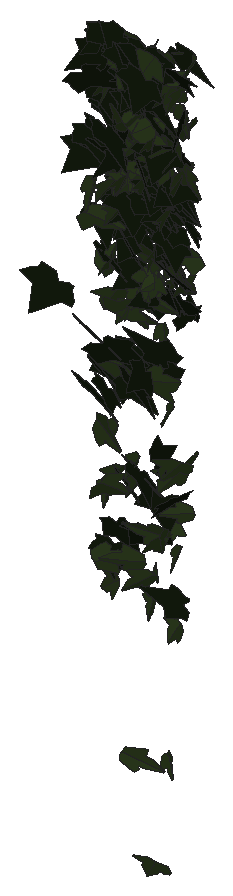
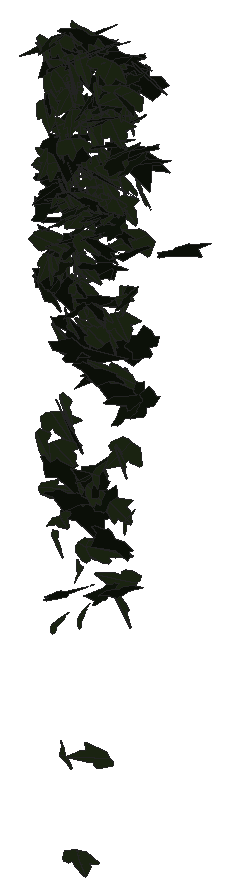
# SketchUp Ruby script. Lengths in millimetres.
U = 1.mm
M = Sketchup.active_model
def pt(a) = Geom::Point3d.new(a.map { |v| v * U })
def face(e, loops, mat)
  f = e.add_face(loops[0].map { |a| pt(a) })
  loops[1..].each { |l| e.add_face(l.map { |a| pt(a) }).erase! }
  f.material = f.back_material = mat if mat
  f
end
# faces: each face lists its corners as indices into pts; further lists are holes
def faces(e, pts, list, mat = nil) = list.each { |f| face(e, (f[0].is_a?(Array) ? f : [f]).map { |l| l.map { |i| pts[i] } }, mat) }
# xy, xz, yz: faces in a plane at the given z, y or x. An outline is a flat list of corners, or four numbers for a rectangle; further outlines are holes
def ring(l) = l.size == 4 ? [[l[0], l[1]], [l[2], l[1]], [l[2], l[3]], [l[0], l[3]]] : l.each_slice(2).to_a
def flat(e, list, mat, &to3) = list.each { |f| face(e, (f[0].is_a?(Array) ? f : [f]).map { |l| ring(l).map { |u, v| to3.(u, v) } }, mat) }
def xy(e, z, list, mat = nil) = flat(e, list, mat) { |x, y| [x, y, z] }
def xz(e, y, list, mat = nil) = flat(e, list, mat) { |x, z| [x, y, z] }
def yz(e, x, list, mat = nil) = flat(e, list, mat) { |y, z| [x, y, z] }
def lines(e, pts, list) = list.each { |a, b| e.add_line(pt(pts[a]), pt(pts[b])) }
# prism: a flat outline (further loops are holes) pulled along v
def prism(e, loops, v, mat = nil)
  f = face(e, loops, mat); d = Geom::Vector3d.new(v.map { |x| x * U })
  f.pushpull(f.normal.samedirection?(d) ? d.length : -d.length)
end
def box(e, o, s, mat = nil) = prism(e, [[o, [o[0] + s[0], o[1], o[2]], [o[0] + s[0], o[1] + s[1], o[2]], [o[0], o[1] + s[1], o[2]]]], [0, 0, s[2]], mat)
def at(x, y, z, deg = 0) = Geom::Transformation.translation(pt([x, y, z])) * Geom::Transformation.rotation(ORIGIN, Z_AXIS, deg.degrees)
def axes(o, x, y, z) = Geom::Transformation.new([*x, 0, *y, 0, *z, 0, *pt(o).to_a, 1])
def part(name) = M.definitions.add(name)
# library, detail: a bought-in or finely detailed component or shape, given as its bounding box
def library(name, o, s) = part(name).tap { |d| box(d.entities, o, s) }
def detail(e, o, s) = box(e.add_group.entities, o, s)
def put(e, d, t, mat = nil) = e.add_instance(d, t).tap { |i| i.material = mat if mat }
def group(e, t, mat = nil) = e.add_group.tap { |g| g.transformation = t; g.material = mat if mat }.entities
root = M.entities
M.materials.add("efeu1").color = [18, 25, 13]
M.materials.add("efeu2").color = [43, 57, 29]
c1 = part("ivyleaf_9")
p = [[39.1,54.8,31.7],[34.5,51.8,30.2],[-5.3,25.2,17.3],[-17.9,28.3,20.9],[-21.6,21.7,17],[-20.2,4.3,5.3],
  [-22.9,-0.3,2.5],[-17.1,-4,-0.6],[-2,-2.1,-1.2],[-0.7,-15.4,-10.1],[16.6,-22.3,-16.7],[21.1,-15.1,-12.5],
  [32.7,-10.7,-11],[46.1,-1.8,-6.6],[30.8,11.2,3.8]]
faces(c1.entities,p,[[0,1,2,3,4,5,6,7,8,9,10,11,12,13,14]],"efeu1")
c2 = part("ivyleaf_10")
p = [[0,12.8,-0.8],[-1.5,51.3,-10.9],[-4.9,51,-11.6],[-13.6,26.5,-7.3],[-13.2,15.9,-4.6],[-21.1,19.3,-7.2],
  [-29.5,16.3,-8.3],[-29.2,8.3,-6.2],[-19.7,-9.8,0.5],[-7.6,-13,4],[1,-12.2,5.8],[-0.4,51.1,-11.1],
  [-1.5,51.1,-10.9],[1,-12.4,5.9],[16.9,-12.4,3.5],[35.1,9.1,-5.1],[35,12.9,-6.1],[20.5,16.4,-4.9],
  [15.8,15,-3.8],[15.3,27.6,-7.1],[12.8,31.3,-7.8]]
faces(c2.entities,p,[[0,1,2,3,4,5,6,7,8,9,10],[11,12,0,13,14,15,16,17,18,19,20]],"efeu2")
put(root,c1,axes([1383.5,966.4,1257.2],[-0.18565,-0.81237,-0.03715],[-0.00199,0.03754,-0.81819],[1.54772,-0.09739,-0.00551]))
put(root,c1,axes([1375.5,982.3,1174.7],[0.78322,-0.66558,-0.0595],[-0.06187,0.04986,-0.78253],[1.27028,0.41281,-0.00143]))
put(root,c2,axes([1392.2,961.8,1154.5],[0.19233,0.43423,-0.7713],[0.2857,0.75665,0.44565],[1.66017,-0.18052,0.01266]))
put(root,c1,axes([1404.6,919.2,1408.9],[-1.08984,-0.55615,0.3063],[-0.4056,-0.22018,-0.79821],[1.13828,-0.61094,0.00884]))
put(root,c1,axes([1401.9,817.4,1189],[-0.98408,-0.7657,0.35319],[-0.37558,-0.29292,-0.92393],[1.56027,-0.55344,0.00036]))
put(root,c1,axes([1390.4,991.5,581.7],[-0.42642,-0.73146,-0.03867],[0.02209,0.03689,-0.76501],[1.39389,-0.22435,0.00029]))
put(root,c1,axes([1381.2,961.4,1429.5],[0.25074,-0.76568,0.26519],[0.03916,-0.26543,-0.77658],[1.54168,0.13127,-0.0234]))
put(root,c1,axes([1413.5,922.4,1607.9],[-1.48911,0.25969,-0.15704],[0.25456,-0.09474,-0.82306],[-0.51847,-0.79239,0.04694]))
put(root,c1,axes([1388.4,976.2,1599.5],[-0.33598,-0.66441,0.46982],[0.06722,-0.48655,-0.6748],[1.54725,-0.12314,0.13134]))
put(root,c2,axes([1403.1,984.2,740.7],[-0.16619,-0.65374,0.43706],[-0.0428,-0.43749,-0.65888],[1.49603,-0.08514,0.0297]))
put(root,c2,axes([1404.7,989.4,1515.6],[-0.62529,-0.70465,0.21746],[-0.00263,-0.23747,-0.7716],[1.40349,-0.31439,0.09544]))
put(root,c2,axes([1403,962.3,1167.3],[0.01424,-0.65222,-0.3851],[0.01668,0.38517,-0.65217],[1.44144,0.00199,0.01135]))
put(root,c1,axes([1386.3,983.2,1464.5],[0.0237,-0.7808,0.15686],[0.08453,-0.15596,-0.77982],[1.51335,0.02094,0.0411]))
put(root,c2,axes([1390.4,970.3,707.1],[-0.11612,-0.33846,0.66501],[0.68804,-0.5971,-0.27073],[1.24234,0.29906,0.21209]))
put(root,c2,axes([1384.8,976.6,1581.2],[-1.09415,-0.2681,-0.53427],[1.02316,0.09222,-0.62475],[0.49743,-0.77939,0.10986]))
put(root,c2,axes([1401.6,954,1527.8],[-0.08183,-0.71014,-0.39764],[0.15773,0.3923,-0.70957],[1.54094,-0.07787,0.05151]))
put(root,c1,axes([1380.6,952.1,962.6],[1.11983,-0.58371,-0.01156],[-0.00828,0.01203,-0.82879],[1.11111,0.58838,0.00548]))
put(root,c1,axes([1421.5,957.3,1591.2],[0.00068,0.82514,0.02135],[-0.27759,0.02107,-0.81216],[-1.54622,-0.00342,0.14581]))
put(root,c2,axes([1414.1,964,1109.5],[-0.74767,-0.6209,0.19031],[-0.12579,-0.18304,-0.73362],[1.22955,-0.39629,0.04067]))
put(root,c2,axes([1388.3,932.7,1268.5],[-0.64985,-0.38676,-0.75955],[1.19277,0.44065,-0.50611],[1.09947,-0.70664,0.10012]))
put(root,c1,axes([1393.6,955.9,1511.8],[0.11622,-0.80177,-0.0838],[0.00596,0.08428,-0.80404],[1.53423,0.06041,0.00947]))
put(root,c1,axes([1380.9,929.1,927.7],[0.64459,-0.71847,0.40917],[0.42658,-0.34582,-0.79277],[1.51466,0.40315,0.04914]))
put(root,c1,axes([1379.7,923.7,1046.8],[0.85251,-0.55382,0.40403],[0.50513,-0.3049,-0.71218],[1.20296,0.52051,0.01272]))
put(root,c2,axes([1417.7,958.3,535.8],[0.71217,-0.58447,-0.45342],[-0.46518,0.3819,-0.694],[1.32877,0.44695,0.00006]))
put(root,c2,axes([1415.4,936.8,1528.4],[0.4615,-0.75581,-0.43029],[-0.22724,0.41354,-0.79368],[1.63957,0.27006,0.01111]))
put(root,c1,axes([1396.2,923.4,1440.7],[-0.05111,-0.77697,-0.22063],[0.04125,0.21998,-0.77732],[1.53665,-0.03175,0.01353]))
put(root,c2,axes([1413.2,962.8,836.9],[0.64822,-0.68731,-0.16805],[-0.09975,0.16149,-0.7667],[1.34293,0.34376,0.02417]))
put(root,c2,axes([1417,947.9,1333.2],[-0.13818,-0.73083,0.2927],[-0.08852,-0.28945,-0.73424],[1.4957,-0.08465,-0.01641]))
put(root,c1,axes([1423.3,914.8,1423],[0.81967,0.40867,-0.6231],[-0.81874,-0.45128,-0.59332],[-1.15799,0.60834,-0.02156]))
put(root,c1,axes([1400.2,960.7,912.8],[-0.01098,-0.62962,0.49023],[0.04838,-0.49014,-0.6292],[1.51791,0.01107,0.0236]))
put(root,c1,axes([1396.8,947.3,1583.9],[1.35766,-0.37155,-0.18742],[-0.17997,0.21749,-0.79108],[0.77128,0.70477,0.14532]))
put(root,c2,axes([1408.9,906.3,1349.8],[0.93175,-0.67898,0.4519],[0.50507,-0.36577,-0.83707],[1.46781,0.55687,0.00117]))
put(root,c1,axes([1397.3,984.5,1311.6],[0.96314,-0.58909,0.01522],[0.01538,-0.01313,-0.77661],[1.12143,0.50612,-0.00243]))
put(root,c1,axes([1406.8,952.5,1495],[-0.02656,-0.78957,0.17307],[-0.0277,-0.17282,-0.78961],[1.53813,-0.01675,-0.01123]))
put(root,c1,axes([1403.9,893.3,1573.3],[-0.03519,0.04954,-0.95837],[0.02758,0.95845,0.04927],[1.8262,-0.01352,-0.01921]))
put(root,c2,axes([1409.1,959.3,1397.8],[1.272,-0.50532,0.29755],[0.42359,-0.19882,-0.83757],[1.03257,0.70406,-0.02296]))
put(root,c1,axes([1437.9,951.7,1630.9],[-1.3885,-0.32156,0.24439],[-0.38375,-0.14723,-0.79565],[0.66604,-0.75519,0.05105]))
put(root,c2,axes([1399.4,949.9,576.1],[0.36962,0.17082,-0.85137],[1.22534,0.55707,0.25864],[1.10893,-0.67248,-0.00201]))
put(root,c1,axes([1407.8,950.8,1634.3],[-0.11101,-0.80044,-0.22127],[0.15875,0.21505,-0.79991],[1.57254,-0.07821,0.06513]))
put(root,c1,axes([1408.7,986.8,1406.1],[0.17531,-0.7858,-0.05674],[-0.00104,0.05706,-0.79115],[1.49942,0.09192,0.00608]))
put(root,c1,axes([1423.3,985,1469.4],[-0.76393,-0.64655,0.26374],[-0.14638,-0.26143,-0.75792],[1.32087,-0.4029,0.06854]))
put(root,c1,axes([1399,976.2,1438.8],[0.97484,-0.5797,0.21818],[0.25307,-0.1736,-0.77343],[1.15136,0.52898,-0.01472]))
put(root,c2,axes([1426.2,976.8,1623],[-1.51465,0.22786,-0.01391],[0.02986,0.00429,-0.82777],[-0.43343,-0.79595,-0.00844]))
put(root,c1,axes([1438.2,967.5,1294.5],[-1.54182,-0.05819,-0.14847],[0.28153,0.01297,-0.8122],[0.11339,-0.82351,-0.0023]))
put(root,c2,axes([1429.2,973.1,1080.6],[0.80247,-0.61306,-0.02625],[-0.01374,0.02689,-0.74401],[1.16777,0.4216,0.00928]))
put(root,c2,axes([1419.7,961.6,1407.7],[-0.37305,-0.80945,0.23875],[0.26558,0.21065,0.82873],[-1.58405,0.22594,0.08272]))
put(root,c2,axes([1437.3,969.2,1342],[-1.42296,0.22882,0.1356],[-0.23313,0.06288,-0.78153],[-0.44933,-0.75726,-0.02392]))
put(root,c2,axes([1439.3,948,1295.3],[-0.19729,-0.72072,0.30819],[-0.11005,-0.30299,-0.72802],[1.48776,-0.11798,-0.01298]))
put(root,c1,axes([1433.8,989.2,1518.9],[-0.77503,-0.65943,0.22641],[0.00689,-0.2642,-0.76297],[1.32692,-0.38379,0.1362]))
put(root,c1,axes([1424,979.1,1323.1],[-0.0649,-0.74925,-0.27158],[0.08543,0.26959,-0.74939],[1.51434,-0.04732,0.03064]))
put(root,c1,axes([1418.5,989.2,563.4],[0.61508,-0.69175,0.08443],[0.071,-0.07576,-0.76352],[1.32441,0.32532,0.00172]))
put(root,c1,axes([1442.1,989.7,1219.9],[-1.05635,-0.5197,-0.00477],[0.00635,0.00341,-0.76037],[0.98912,-0.55505,-0.00021]))
put(root,c1,axes([1431.3,958.3,968.4],[-1.04311,-0.38741,-0.45292],[0.77676,0.20444,-0.66876],[0.82662,-0.68098,0.05689]))
put(root,c2,axes([1436.5,967.7,1339.1],[1.1202,0.51681,-0.1362],[-0.18835,-0.0937,-0.78326],[-0.99959,0.59683,-0.00504]))
put(root,c1,axes([1469.6,981.4,1398.5],[-1.24986,0.35112,0.29934],[-0.64225,-0.0104,-0.72813],[-0.59887,-0.72165,0.15615]))
put(root,c2,axes([1450.7,971.8,1419],[-0.7007,-0.65439,0.27216],[-0.12306,-0.2744,-0.74724],[1.34323,-0.3665,0.07352]))
put(root,c1,axes([1429.8,971.7,1535.8],[-0.15257,-0.68111,0.44747],[0.2011,-0.45453,-0.67292],[1.53793,-0.00814,0.13238]))
put(root,c2,axes([1429.8,965.9,1075.1],[-1.17467,-0.4492,0.47082],[0.71501,0.28387,0.76333],[-1.01122,0.72252,-0.00719]))
put(root,c1,axes([1455,994.9,1149.8],[-1.07161,-0.4476,0.28525],[-0.38444,-0.20385,-0.7186],[0.93414,-0.59737,0.03149]))
put(root,c2,axes([1413.7,946.1,980.2],[0.10679,-0.03226,-0.86542],[1.58354,-0.23853,0.06284],[-0.45716,-0.83379,0.01551]))
put(root,c1,axes([1429.3,955.5,654.2],[-0.54245,-0.09388,-0.70569],[1.26493,0.23729,-0.30001],[0.4855,-0.72314,-0.00683]))
put(root,c1,axes([1430.4,973.5,733.9],[0.16223,-0.47252,0.60804],[0.28269,-0.59018,-0.47946],[1.43805,0.16932,0.02566]))
put(root,c1,axes([1464.3,991.5,1263.4],[-1.54721,-0.15313,-0.03686],[0.07134,0.00013,-0.82722],[0.29115,-0.81379,0.0068]))
put(root,c2,axes([1454.9,938.8,1361.2],[-0.04586,-0.79406,-0.01036],[0.00007,0.01036,-0.79442],[1.51138,-0.0241,-0.00028]))
put(root,c1,axes([1425.6,971.8,1222.1],[0.45769,-0.05898,-0.8232],[1.46631,-0.29137,0.24595],[-0.56316,-0.8066,-0.02865]))
put(root,c2,axes([1451.6,970.2,1345.4],[0.2024,-0.70765,0.32439],[0.21977,-0.30944,-0.71289],[1.46517,0.14417,0.06212]))
put(root,c2,axes([1462.4,953.6,1356.1],[-0.65566,-0.57467,0.50948],[-0.17857,-0.52271,-0.65304],[1.45069,-0.32407,0.14988]))
put(root,c1,axes([1456.5,970.9,1492.5],[-0.6835,-0.55118,0.48288],[-0.34395,-0.45452,-0.65322],[1.35155,-0.39441,0.07796]))
put(root,c1,axes([1449.4,980.5,1002.3],[-1.06445,-0.37036,-0.39864],[0.67013,0.18952,-0.67007],[0.78955,-0.66016,0.03128]))
put(root,c1,axes([1434.9,913.1,1031.9],[-0.06917,-0.04612,-0.91215],[0.5345,0.86808,-0.05508],[1.65401,-0.28245,-0.02034]))
put(root,c1,axes([1449.7,984.5,1274.2],[-0.33101,-0.77302,0.05514],[-0.00945,-0.0554,-0.79231],[1.47493,-0.17384,0.0073]))
put(root,c2,axes([1460.8,962.7,1558],[0.21322,-0.81799,-0.13795],[0.03213,0.14143,-0.82487],[1.57846,0.10762,0.03542]))
put(root,c2,axes([1453.6,972.3,781.9],[0.0192,-0.38628,0.67921],[0.42179,-0.64996,-0.37293],[1.42603,0.19744,0.10116]))
put(root,c2,axes([1477.3,906.4,1493.8],[-0.98023,0.32118,0.63002],[-1.00665,0.34237,-0.60694],[-0.89334,-0.73823,-0.00738]))
put(root,c1,axes([1437.2,984.1,1320.6],[0.28187,-0.75304,0.17605],[0.42696,-0.12971,-0.74354],[1.40854,0.19001,0.19015]))
put(root,c2,axes([1461.8,976.2,750.6],[-0.00776,-0.68886,0.41079],[0.03039,-0.41078,-0.68869],[1.52615,0.00468,0.0158]))
put(root,c2,axes([1454.7,975.6,1126],[1.32488,-0.36812,0.07239],[0.1193,-0.03632,-0.78747],[0.70399,0.69894,-0.00279]))
put(root,c1,axes([1436.2,939.2,1543],[0.76918,0.73771,-0.2474],[0.23254,0.21515,0.84115],[1.46248,-0.4222,-0.00363]))
put(root,c2,axes([1468.4,992.8,1267.4],[-0.46568,-0.60599,0.41848],[-0.13139,-0.42016,-0.64878],[1.39543,-0.24179,0.07857]))
put(root,c2,axes([1482.8,937.3,607.9],[-0.08652,-0.04195,0.78348],[-0.90717,-0.6219,-0.06095],[1.18611,-0.4787,0.01053]))
put(root,c2,axes([1483.1,988,1339.9],[-1.00138,-0.09019,0.55147],[-0.75997,-0.46919,-0.45772],[0.74397,-0.60069,0.27472]))
put(root,c2,axes([1440.6,983.9,1068.2],[-0.61494,-0.11608,0.7013],[1.33211,-0.18639,0.29163],[0.2361,0.74932,0.18118]))
put(root,c2,axes([1467.2,966.2,1469.8],[0.2262,-0.79103,0.21126],[0.10431,-0.20531,-0.79958],[1.55476,0.12886,0.02291]))
put(root,c1,axes([1453.9,930.4,1447.5],[0.06453,0.2424,0.91267],[-0.11875,-0.91069,0.24419],[1.79329,-0.06903,-0.01667]))
put(root,c2,axes([1466.4,963.3,1374.5],[0.74133,0.64995,-0.26409],[-0.28313,-0.21867,-0.7576],[-1.30483,0.41671,0.01435]))
put(root,c1,axes([1479.4,895.2,1436.2],[-1.25679,0.45424,-0.35024],[0.56807,-0.18394,-0.80134],[-0.9322,-0.7245,-0.01614]))
put(root,c1,axes([1456.2,981.6,1511.3],[0.31894,-0.77335,-0.15333],[-0.06192,0.14984,-0.7913],[1.49922,0.17071,-0.00006]))
put(root,c2,axes([1491.9,972.8,1199.9],[0.48907,-0.07163,-0.74482],[-1.01523,0.53472,-0.23547],[0.99865,0.57867,0.12538]))
put(root,c1,axes([1449,977.7,759.9],[0.47248,-0.48225,0.58906],[0.4952,-0.52853,-0.54235],[1.36163,0.35956,-0.00716]))
put(root,c1,axes([1467.6,973.8,1114],[-0.73976,0.47204,0.48785],[0.41249,-0.44645,0.60466],[1.22434,0.43562,0.09105]))
put(root,c1,axes([1455.4,891.2,1477.8],[0.41536,-0.93251,0.16658],[0.082,-0.161,-0.95769],[1.80097,0.22239,0.00518]))
put(root,c1,axes([1471.3,942.8,1320.6],[-0.74891,-0.6556,-0.22542],[0.23136,0.18994,-0.7646],[1.299,-0.4118,0.00622]))
put(root,c2,axes([1481.3,948.1,1488],[-0.02365,-0.86291,0.05121],[-0.00567,-0.05118,-0.86299],[1.64516,-0.01258,-0.00224]))
put(root,c2,axes([1470.3,868.4,787.4],[-0.64382,-0.54157,-0.74252],[0.67827,0.65201,-0.63792],[1.61226,-0.49056,-0.02814]))
put(root,c1,axes([1465.9,993.6,1289.5],[-0.0201,-0.67299,0.37796],[0.04028,-0.3781,-0.67266],[1.46845,0.00116,0.02362]))
put(root,c2,axes([1483.6,980.2,1614.3],[-0.08397,-0.82303,-0.06945],[-0.05042,0.07093,-0.82366],[1.57115,-0.04171,-0.03015]))
put(root,c1,axes([1480.1,989.7,1340.6],[-1.19984,-0.30698,-0.31151],[0.50774,0.16312,-0.70067],[0.65956,-0.68401,-0.02729]))
put(root,c2,axes([1472.8,994.7,499.3],[-0.11947,-0.3232,0.67328],[0.65692,-0.61172,-0.26147],[1.26047,0.28818,0.20008]))
put(root,c2,axes([1458.3,954.2,200.6],[0.40501,0.14576,0.7096],[1.11876,0.39748,-0.25794],[-0.80574,0.62516,-0.00146]))
put(root,c1,axes([1465.8,981.7,1333.4],[0.58645,-0.72164,0.06926],[0.03261,-0.06799,-0.7846],[1.37935,0.30842,-0.0109]))
put(root,c1,axes([1467,934.7,1622.4],[0.66084,-0.76942,-0.06184],[-0.04143,0.05802,-0.84413],[1.4685,0.34788,0.00401]))
put(root,c1,axes([1486.6,989.7,1115.7],[0.28783,-0.46828,-0.67227],[0.39805,-0.63891,0.49209],[-1.5076,-0.25809,0.00158]))
put(root,c1,axes([1480.2,924.3,1617.9],[-0.49893,-0.79199,0.19051],[-0.0126,-0.19805,-0.83246],[1.55026,-0.2565,0.05455]))
put(root,c2,axes([1488.9,920,1603],[1.77113,-0.20864,-0.13188],[-0.24083,0.03838,-0.95366],[0.40332,0.93912,0.00968]))
put(root,c2,axes([1500.8,968.8,-5.7],[-1.1786,-0.10255,0.21179],[-0.39254,-0.05045,-0.62752],[0.21557,-0.65254,0.01524]))
put(root,c1,axes([1476.3,929.4,968],[0.23842,-0.60232,-0.53817],[-0.05169,0.54115,-0.61198],[1.53639,0.11168,0.06293]))
put(root,c1,axes([1481.2,962.1,1526.1],[0.8051,-0.53796,-0.47731],[-0.60686,0.35606,-0.68391],[1.22687,0.52915,-0.02506]))
put(root,c1,axes([1476.9,958.3,772.2],[0.13694,-0.77133,0.35049],[0.07731,-0.34821,-0.77464],[1.61059,0.0823,0.00738]))
put(root,c2,axes([1502,980.5,1438],[-1.12114,-0.51571,0.21154],[-0.20008,-0.19947,-0.77903],[1.04183,-0.59328,0.07803]))
put(root,c2,axes([1492.9,979.8,1210.4],[0.32863,-0.71806,0.19471],[0.14421,-0.18187,-0.73791],[1.4086,0.18615,0.03012]))
put(root,c2,axes([1463,863,902.8],[0.31688,-0.09511,0.96969],[1.6343,-0.45051,-0.19163],[0.87621,0.87468,0.00674]))
put(root,c2,axes([1488.8,978.6,1305.3],[-1.39728,0.25942,-0.19684],[0.35141,-0.06827,-0.77865],[-0.51051,-0.75703,0.00276]))
put(root,c2,axes([1498.8,946.5,1372.3],[0.01417,-0.79412,-0.10304],[-0.00905,0.103,-0.79414],[1.52401,0.00799,-0.00376]))
put(root,c2,axes([1490.3,971.3,1157.9],[1.39277,-0.31697,0.05665],[0.09934,-0.02203,-0.7975],[0.60472,0.73366,0.00053]))
put(root,c1,axes([1481.7,986.9,1329.8],[0.12256,-0.73438,0.20839],[0.0279,-0.2079,-0.73719],[1.45259,0.06596,-0.00342]))
put(root,c1,axes([1483.8,962.9,1618.6],[-0.10741,-0.83909,0.0994],[0.01669,-0.1002,-0.84084],[1.60803,-0.05501,0.01537]))
put(root,c2,axes([1497.9,979.6,1155.2],[-0.41985,-0.06764,0.72159],[0.18668,-0.75013,-0.04033],[1.36667,0.08168,0.22719]))
put(root,c2,axes([1494.4,978.7,575.7],[-0.05844,0.2233,-0.60377],[-0.01288,-0.60453,-0.22324],[-1.2251,-0.0043,0.03115]))
put(root,c1,axes([1478.9,979.3,1585.9],[0.41739,-0.75212,-0.27112],[0.15855,0.3011,-0.76791],[1.51332,0.17589,0.15523]))
put(root,c1,axes([1530.3,953.3,1595.3],[-1.2615,0.12822,0.51203],[-0.97317,0.048,-0.67394],[-0.24929,-0.83619,0.03983]))
put(root,c1,axes([1513,936.6,679.8],[0.61472,0.46235,-0.55271],[-0.66271,-0.43013,-0.5633],[-1.20068,0.47412,0.02794]))
put(root,c2,axes([1504.7,982.3,1595.7],[0.77483,-0.68811,-0.19455],[-0.02513,0.2166,-0.79373],[1.36072,0.39583,0.09612]))
put(root,c1,axes([1537.2,949.4,989.2],[-0.43877,0.07388,0.8996],[-1.6997,0.11607,-0.2384],[-0.24929,-0.92139,0.0421]))
put(root,c1,axes([1490.8,979.4,1366.7],[0.35715,-0.75026,-0.16423],[-0.08833,0.15767,-0.77335],[1.45904,0.1932,-0.00662]))
put(root,c2,axes([1501.8,982.5,1497.8],[-0.16209,-0.81874,-0.02947],[0.41366,0.00599,-0.79447],[1.50336,-0.08992,0.21542]))
put(root,c2,axes([1477.9,973.5,1118.1],[-0.27444,0.00621,-0.78452],[1.37287,-0.31259,-0.13506],[-0.5871,-0.73386,0.05089]))
put(root,c2,axes([1508.4,976.2,1390.2],[0.39027,-0.77516,0.02329],[-0.00521,-0.02481,-0.80178],[1.47594,0.20488,-0.00899]))
put(root,c2,axes([1518.6,924.5,593.2],[-0.34375,-0.49797,0.59155],[-0.39999,-0.55299,-0.52968],[1.41623,-0.27705,-0.00602]))
put(root,c1,axes([1502.4,974.9,1344.5],[-0.59711,-0.68993,0.23057],[0.05964,-0.26368,-0.74639],[1.38318,-0.28647,0.13172]))
put(root,c2,axes([1527,954.7,1399.1],[0.49779,-0.2663,-0.76266],[-0.94843,0.57774,-0.37264],[1.21003,0.56239,0.02167]))
put(root,c1,axes([1490.6,986.2,1318.9],[0.49213,-0.71561,0.19912],[0.13839,-0.18544,-0.76087],[1.40689,0.26856,0.00519]))
put(root,c2,axes([1515.6,962.8,1208.8],[0.52546,-0.54792,-0.48432],[-0.12415,0.49717,-0.59965],[1.38624,0.25222,0.12988]))
put(root,c1,axes([1494,952.8,1330.7],[0.2059,-0.64098,-0.45302],[0.24989,0.46563,-0.62747],[1.47278,0.01061,0.1698]))
put(root,c1,axes([1516.7,975.6,1428.8],[1.23403,0.20638,-0.50511],[-0.91581,-0.15359,-0.68045],[-0.48961,0.80745,-0.00033]))
put(root,c2,axes([1540.4,932.3,681.1],[-0.39451,0.04473,-0.76954],[-1.42273,-0.20609,0.18938],[-0.35794,0.76986,0.09541]))
put(root,c2,axes([1490,932.9,1470.9],[1.2301,0.15459,-0.64452],[1.1537,0.22614,0.66214],[0.51007,-0.88431,0.05666]))
put(root,c2,axes([1521.6,955.9,1418.6],[-0.73764,-0.69551,0.15029],[-0.03526,-0.16121,-0.79386],[1.35379,-0.38317,0.06121]))
put(root,c1,axes([1507,990.3,1288.8],[-0.21872,-0.66719,0.38842],[0.01283,-0.39356,-0.67401],[1.46924,-0.09588,0.06371]))
put(root,c2,axes([1520.4,937,1463.5],[-0.02483,-0.75711,-0.35889],[0.00278,0.35891,-0.75721],[1.59462,-0.01241,-0.00427]))
put(root,c1,axes([1544,942.8,1029.9],[-0.15705,0.05785,0.78716],[-1.1823,0.48346,-0.10065],[-0.92663,-0.62665,-0.00499]))
put(root,c1,axes([1496.5,910.9,987.2],[0.52383,-0.8008,0.36856],[0.20139,-0.3533,-0.84667],[1.66561,0.29457,-0.01354]))
put(root,c2,axes([1520.7,982.6,1340.6],[0.79327,-0.66314,-0.05401],[-0.04071,0.05034,-0.7832],[1.26561,0.41727,0.00866]))
put(root,c1,axes([1505.7,927.6,1633.3],[-0.88666,-0.49417,-0.62927],[0.87965,0.42817,-0.67843],[1.243,-0.65551,0.03124]))
put(root,c1,axes([1512.8,925.2,1000.8],[0.35838,-0.35523,-0.79583],[0.8013,-0.6758,0.40127],[-1.45227,-0.46054,0.02502]))
put(root,c1,axes([1505.7,995.1,1195.5],[0.18701,-0.67145,0.35087],[0.05647,-0.35013,-0.67833],[1.44075,0.10088,-0.01896]))
put(root,c1,axes([1521.2,992.6,1239.7],[-0.69728,-0.59287,0.32661],[-0.17918,-0.32314,-0.69218],[1.27572,-0.36944,0.0813]))
put(root,c1,axes([1508.5,987.3,1327.8],[-0.03666,-0.76026,0.19273],[0.04456,-0.19326,-0.76001],[1.49204,-0.01291,0.02743]))
put(root,c1,axes([1514.1,977.4,724.2],[-0.84004,-0.52209,-0.37281],[0.44326,0.29124,-0.6836],[1.13765,-0.49898,-0.00893]))
put(root,c2,axes([1523.8,960.2,1565.3],[0.42794,-0.77012,-0.20303],[-0.02112,0.20792,-0.80095],[1.51563,0.22034,0.04617]))
put(root,c2,axes([1529.2,966.3,1310],[-0.88981,-0.60687,0.21071],[-0.13219,-0.21132,-0.76275],[1.21546,-0.46725,0.0713]))
put(root,c1,axes([1506.6,950.5,1502.7],[1.14192,-0.53386,-0.38343],[-0.47458,0.29547,-0.80159],[1.15743,0.64786,0.04962]))
put(root,c2,axes([1516.1,971.8,1532.7],[-0.41858,-0.6912,-0.40577],[0.52072,0.33075,-0.71171],[1.4338,-0.32191,0.14002]))
put(root,c1,axes([1530.5,937.2,1618.1],[-1.1156,0.35221,-0.49475],[0.72872,-0.31941,-0.68103],[-0.89718,-0.69739,0.06205]))
put(root,c1,axes([1539.7,992.1,516],[-0.34916,-0.71733,-0.2546],[-0.12596,-0.24587,0.74041],[-1.44317,0.19501,-0.00303]))
put(root,c2,axes([1528.1,975.2,906.9],[0.36705,-0.77536,-0.08895],[-0.06006,0.08381,-0.79892],[1.48414,0.19515,-0.01033]))
put(root,c2,axes([1529.5,956.7,1576.6],[1.11759,0.59892,0.13219],[-0.18399,-0.09034,0.83874],[1.1527,-0.59509,0.00571]))
put(root,c2,axes([1529.2,977.7,1375.5],[0.87748,-0.66138,-0.1514],[-0.10296,0.14663,-0.80529],[1.28718,0.46259,0.03879]))
put(root,c2,axes([1529,916.6,1630.1],[1.55988,-0.50896,-0.13471],[-0.2183,0.07064,-0.96478],[0.97794,0.8276,-0.00049]))
put(root,c2,axes([1540.8,957.2,1557.4],[-1.28912,-0.4383,0.27879],[-0.41772,-0.17374,-0.80639],[0.89604,-0.71157,0.02516]))
put(root,c2,axes([1534.2,978.3,1567.4],[-0.28163,-0.69496,0.40224],[-0.10952,-0.39878,-0.71016],[1.52428,-0.15706,0.02329]))
put(root,c2,axes([1531.5,965.6,1426],[-0.25156,-0.76363,0.2853],[0.04403,-0.29242,-0.77198],[1.55084,-0.11557,0.06819]))
put(root,c2,axes([1512.2,989.3,200.7],[0.54195,-0.25308,0.5701],[0.83153,-0.36634,-0.38086],[0.84724,0.52144,0.00913]))
put(root,c2,axes([1531.2,951.1,1546.8],[0.1779,-0.81307,-0.20921],[0.00754,0.21093,-0.81798],[1.59782,0.08953,0.02715]))
put(root,c1,axes([1539.3,975.6,1316.9],[-0.97418,-0.41326,0.42393],[-0.49362,-0.34723,-0.65166],[1.01286,-0.5667,0.09015]))
put(root,c1,axes([1527.7,956.6,1434.3],[-0.8477,-0.69657,-0.01807],[0.01176,0.01749,-0.82679],[1.3261,-0.44543,-0.00422]))
put(root,c1,axes([1511.2,938.8,1548.5],[0.77497,-0.80713,-0.17965],[-0.15992,0.15883,-0.90402],[1.56557,0.41576,-0.00341]))
put(root,c2,axes([1515.5,970.7,1066.4],[0.71583,-0.3326,0.5645],[0.78353,-0.38638,-0.50196],[0.97006,0.55752,-0.01112]))
put(root,c2,axes([1531.9,979.9,673.7],[0.40159,0.533,-0.30857],[-0.28051,-0.273,-0.57234],[-1.13808,0.25537,0.03218]))
put(root,c1,axes([1534.1,977.6,1345.2],[-0.49196,-0.45142,0.61389],[-0.34847,-0.59247,-0.51276],[1.40776,-0.30441,0.08761]))
put(root,c1,axes([1515.7,969.1,1224.5],[1.02517,-0.57731,-0.10779],[-0.1438,0.07693,-0.78957],[1.10843,0.54392,-0.00274]))
put(root,c2,axes([1529,995.6,464.9],[-0.40066,-0.17023,0.70196],[0.49112,-0.70064,-0.09252],[1.28398,0.21488,0.25443]))
put(root,c2,axes([1540.2,984.1,1561.5],[-0.57288,-0.75399,0.07161],[-0.02875,-0.07107,-0.81176],[1.44116,-0.30114,0.01227]))
put(root,c1,axes([1520.6,949,814.9],[-0.12102,0.53229,0.76026],[0.14748,-0.75634,0.53602],[1.76015,0.09997,0.00736]))
put(root,c1,axes([1537.3,972.5,1275.3],[-0.8386,-0.63039,0.10894],[-0.09357,-0.09852,-0.76895],[1.21394,-0.44307,0.01599]))
put(root,c2,axes([1539.1,966.8,1414.7],[0.35779,-0.79558,-0.04818],[-0.02323,0.04662,-0.81749],[1.51674,0.18839,-0.00116]))
put(root,c2,axes([1539.7,964.8,1206.9],[0.8173,-0.58418,-0.29455],[-0.15601,0.30151,-0.7175],[1.23532,0.42458,0.10426]))
put(root,c2,axes([1543.2,965.1,1623.2],[-0.46244,-0.78326,0.17958],[0.04315,-0.19422,-0.81642],[1.52877,-0.23145,0.07737]))
put(root,c2,axes([1548.4,963.6,1456.4],[0.94752,-0.40858,-0.48347],[-0.29742,0.51671,-0.5976],[1.16742,0.46326,0.24015]))
put(root,c1,axes([1526.2,963.2,1335.5],[-0.17347,-0.2557,-0.77693],[0.41246,0.74625,-0.27103],[1.50105,-0.23461,-0.01531]))
put(root,c2,axes([1540.8,982.8,626.1],[0.62081,-0.64833,0.21678],[0.19832,-0.19024,-0.72573],[1.28586,0.34236,0.00727]))
put(root,c1,axes([1548,983.8,1363.3],[-1.01627,-0.57417,0.07972],[-0.09596,-0.06197,-0.78408],[1.09906,-0.53633,0.00525]))
put(root,c1,axes([1539.8,889.3,1606.9],[-0.51288,-0.81812,0.36655],[-0.16586,-0.35704,-0.86095],[1.69811,-0.28197,0.02662]))
put(root,c1,axes([1563.2,963.3,1145.4],[0.61609,0.19882,-0.72635],[-1.3329,-0.21114,-0.36992],[-0.52685,0.76668,0.08649]))
put(root,c2,axes([1549.9,975.2,1184.7],[0.0677,-0.76413,0.08481],[0.00969,-0.08467,-0.76495],[1.46318,0.03592,0.00114]))
put(root,c2,axes([1555.9,956.7,796.3],[-0.67238,-0.5784,0.42474],[-0.19188,-0.42872,-0.66768],[1.35219,-0.34845,0.11646]))
put(root,c2,axes([1571.9,981.4,1225.6],[0.63854,0.01484,-0.73285],[-1.38688,-0.08035,-0.33524],[-0.15077,0.80199,-0.02002]))
put(root,c1,axes([1537,952.3,1600.6],[1.58018,0.05338,-0.16893],[-0.32395,0.0158,-0.83158],[-0.09352,0.84714,0.02616]))
put(root,c2,axes([1553.3,940,1326.9],[0.14959,-0.7876,0.0599],[0.02037,-0.05913,-0.7915],[1.50316,0.07918,0.00477]))
put(root,c1,axes([1538.4,982.6,1346.9],[0.35258,-0.66908,-0.41049],[-0.2079,0.39569,-0.69426],[1.47942,0.21506,0.00026]))
put(root,c2,axes([1542,971.2,1212.7],[-0.52952,0.54544,-0.51617],[0.41112,-0.46906,-0.6121],[-1.36881,-0.35189,0.01584]))
put(root,c1,axes([1544.3,964.6,1258.1],[-0.22481,-0.78423,0.15144],[0.02046,-0.15464,-0.79239],[1.51998,-0.11391,0.03306]))
put(root,c2,axes([1567.8,973.4,717],[-0.20577,0.0104,0.6499],[-0.49349,-0.60483,-0.03346],[1.13436,-0.26123,0.10333]))
put(root,c2,axes([1557.2,976,1183.8],[0.74742,-0.53614,-0.38819],[-0.04378,0.44005,-0.63103],[1.25901,0.33359,0.20851]))
put(root,c1,axes([1536.6,973.1,1149.2],[0.59981,-0.19048,-0.71429],[1.12313,-0.40285,0.36781],[-0.84739,-0.66877,-0.01811]))
put(root,c1,axes([1569,941.6,759.5],[-0.31795,0.76038,-0.38991],[0.16387,-0.38029,-0.77851],[-1.61804,-0.18793,-0.00223]))
put(root,c2,axes([1558.1,968,1553.7],[0.20598,-0.68902,0.4656],[0.10461,-0.46257,-0.69732],[1.57921,0.12051,-0.01454]))
put(root,c2,axes([1560.8,959.7,1383.7],[0.30231,-0.77836,-0.1545],[-0.02304,0.15517,-0.79418],[1.5101,0.15819,0.01881]))
put(root,c2,axes([1533.5,932.1,984.9],[0.8284,-0.32687,-0.74749],[1.09351,-0.47865,0.54389],[-1.10231,-0.72048,-0.0222]))
put(root,c2,axes([1559.7,974.6,1393.5],[-0.24962,-0.67818,-0.52389],[0.37539,0.49187,-0.68611],[1.58718,-0.22299,0.07988]))
put(root,c2,axes([1567.9,976.7,1490.7],[-0.32009,-0.79744,-0.10396],[-0.00056,0.10627,-0.81469],[1.53054,-0.16674,-0.02204]))
put(root,c1,axes([1542.3,872.3,1448.1],[0.28181,-0.04382,-0.8756],[1.4564,-0.42684,0.15077],[-0.81415,-0.77872,-0.03337]))
put(root,c2,axes([1567.1,896.8,698.7],[-0.26498,-0.78876,-0.40578],[0.17044,0.39615,-0.80077],[1.67955,-0.16464,0.01724]))
put(root,c2,axes([1551.1,984.5,1388.7],[-0.8188,0.49222,-0.54563],[0.69516,-0.40538,-0.65371],[-1.21355,-0.56433,-0.00632]))
put(root,c1,axes([1579.8,961.5,1113.2],[-0.86104,0.41044,-0.53673],[-0.74537,0.36708,0.61082],[1.04791,0.59835,-0.00655]))
put(root,c1,axes([1548.2,978.3,1628.9],[0.86394,-0.64181,-0.28018],[-0.0859,0.30638,-0.77497],[1.33004,0.43668,0.13194]))
put(root,c2,axes([1582.1,931.9,835.5],[-0.92265,-0.55595,0.32133],[-0.41101,-0.23802,-0.73761],[1.15092,-0.53068,-0.00581]))
put(root,c1,axes([1544.6,950.7,1196.9],[0.20658,-0.43292,0.64366],[0.72977,-0.53502,-0.42452],[1.28333,0.37393,0.13779]))
put(root,c2,axes([1568.8,968.9,1175.8],[-0.2964,-0.60785,-0.51435],[0.28192,0.49283,-0.62727],[1.48899,-0.21431,0.01638]))
put(root,c1,axes([1552.6,991.8,1288.6],[0.18173,-0.5978,0.53452],[0.19821,-0.5245,-0.60519],[1.5133,0.14049,0.01508]))
put(root,c2,axes([1571.9,986.4,821.2],[0.25081,-0.77373,0.16641],[0.05128,-0.16421,-0.78487],[1.50535,0.13451,-0.00099]))
put(root,c2,axes([1557.5,973.8,1516.1],[0.89418,-0.54733,0.40577],[0.77871,-0.16747,-0.69964],[1.03686,0.59778,0.17552]))
put(root,c2,axes([1575.2,978.8,1616.1],[0.42395,-0.79275,0.05545],[0.01421,-0.05549,-0.82341],[1.51237,0.22274,-0.0078]))
put(root,c1,axes([1569.1,964.4,1511.5],[-0.39541,0.21973,-0.78211],[1.06265,-0.54777,-0.30221],[-1.12308,-0.59566,-0.01059]))
